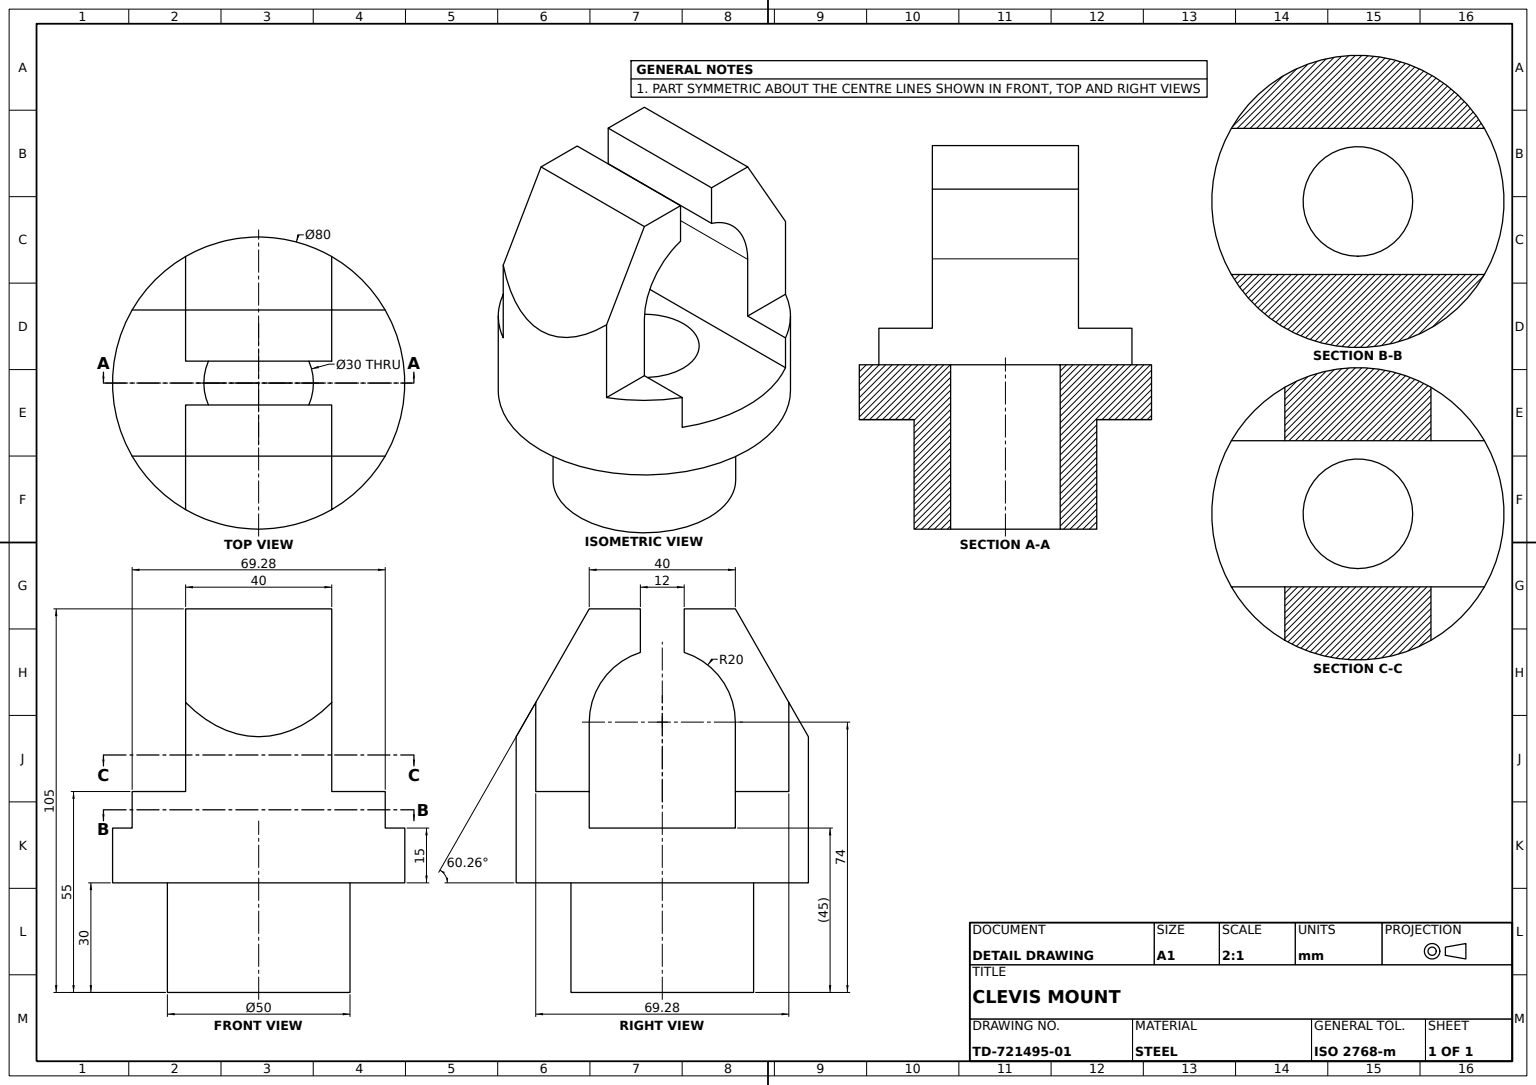
ISO-10303-21;
HEADER;
FILE_DESCRIPTION((''),'2;1');
FILE_NAME('','',(''),(''),'','','');
FILE_SCHEMA(('AUTOMOTIVE_DESIGN'));
ENDSEC;
DATA;
#1=APPLICATION_CONTEXT('');
#2=PRODUCT_CONTEXT('',#1,'mechanical');
#3=PRODUCT('','','',(#2));
#4=PRODUCT_DEFINITION_FORMATION('','',#3);
#5=PRODUCT_DEFINITION_CONTEXT('',#1,'design');
#6=PRODUCT_DEFINITION('','',#4,#5);
#7=PRODUCT_DEFINITION_SHAPE('','',#6);
#8=(LENGTH_UNIT()NAMED_UNIT(*)SI_UNIT(.MILLI.,.METRE.));
#9=(NAMED_UNIT(*)PLANE_ANGLE_UNIT()SI_UNIT($,.RADIAN.));
#10=(NAMED_UNIT(*)SI_UNIT($,.STERADIAN.)SOLID_ANGLE_UNIT());
#11=UNCERTAINTY_MEASURE_WITH_UNIT(LENGTH_MEASURE(0.005),#8,'distance_accuracy_value','');
#12=(GEOMETRIC_REPRESENTATION_CONTEXT(3)GLOBAL_UNCERTAINTY_ASSIGNED_CONTEXT((#11))GLOBAL_UNIT_ASSIGNED_CONTEXT((#8,#9,#10))REPRESENTATION_CONTEXT('',''));
#13=CARTESIAN_POINT('',(20.,34.641016,79.378222));
#14=VERTEX_POINT('',#13);
#15=CARTESIAN_POINT('',(20.,20.,105.));
#16=VERTEX_POINT('',#15);
#17=CARTESIAN_POINT('',(20.,60.307692,34.461538));
#18=DIRECTION('',(0.,-0.496138938,0.868243142));
#19=VECTOR('',#18,1000.);
#20=LINE('',#17,#19);
#21=EDGE_CURVE('',#14,#16,#20,.T.);
#22=ORIENTED_EDGE('',*,*,#21,.F.);
#23=CARTESIAN_POINT('',(-20.,34.641016,79.378222));
#24=VERTEX_POINT('',#23);
#25=CARTESIAN_POINT('',(0.,0.,140.));
#26=DIRECTION('',(0.,-0.868243142,-0.496138938));
#27=DIRECTION('',(0.,0.496138938,-0.868243142));
#28=AXIS2_PLACEMENT_3D('',#25,#26,#27);
#29=ELLIPSE('',#28,80.622577,40.);
#30=EDGE_CURVE('',#14,#24,#29,.F.);
#31=ORIENTED_EDGE('',*,*,#30,.T.);
#32=CARTESIAN_POINT('',(-20.,20.,105.));
#33=VERTEX_POINT('',#32);
#34=CARTESIAN_POINT('',(-20.,60.307692,34.461538));
#35=LINE('',#34,#19);
#36=EDGE_CURVE('',#24,#33,#35,.T.);
#37=ORIENTED_EDGE('',*,*,#36,.T.);
#38=CARTESIAN_POINT('',(50.,20.,105.));
#39=DIRECTION('',(-1.,0.,0.));
#40=VECTOR('',#39,1000.);
#41=LINE('',#38,#40);
#42=EDGE_CURVE('',#16,#33,#41,.T.);
#43=ORIENTED_EDGE('',*,*,#42,.F.);
#44=EDGE_LOOP('',(#22,#31,#37,#43));
#45=FACE_BOUND('',#44,.T.);
#46=CARTESIAN_POINT('',(50.,40.,70.));
#47=AXIS2_PLACEMENT_3D('',#46,#26,#27);
#48=PLANE('',#47);
#49=ADVANCED_FACE('',(#45),#48,.F.);
#50=CARTESIAN_POINT('',(34.641016,-20.,45.));
#51=VERTEX_POINT('',#50);
#52=CARTESIAN_POINT('',(34.641016,-20.,55.));
#53=VERTEX_POINT('',#52);
#54=CARTESIAN_POINT('',(34.641016,-20.,105.));
#55=DIRECTION('',(0.,0.,-1.));
#56=VECTOR('',#55,1000.);
#57=LINE('',#54,#56);
#58=EDGE_CURVE('',#51,#53,#57,.F.);
#59=ORIENTED_EDGE('',*,*,#58,.F.);
#60=CARTESIAN_POINT('',(-34.641016,-20.,45.));
#61=VERTEX_POINT('',#60);
#62=CARTESIAN_POINT('',(70.,-20.,45.));
#63=LINE('',#62,#40);
#64=EDGE_CURVE('',#61,#51,#63,.F.);
#65=ORIENTED_EDGE('',*,*,#64,.F.);
#66=CARTESIAN_POINT('',(-34.641016,-20.,55.));
#67=VERTEX_POINT('',#66);
#68=CARTESIAN_POINT('',(-34.641016,-20.,105.));
#69=LINE('',#68,#56);
#70=EDGE_CURVE('',#67,#61,#69,.T.);
#71=ORIENTED_EDGE('',*,*,#70,.F.);
#72=CARTESIAN_POINT('',(-20.,-20.,55.));
#73=VERTEX_POINT('',#72);
#74=CARTESIAN_POINT('',(70.,-20.,55.));
#75=DIRECTION('',(1.,0.,0.));
#76=VECTOR('',#75,1000.);
#77=LINE('',#74,#76);
#78=EDGE_CURVE('',#67,#73,#77,.T.);
#79=ORIENTED_EDGE('',*,*,#78,.T.);
#80=CARTESIAN_POINT('',(-20.,-20.,74.));
#81=VERTEX_POINT('',#80);
#82=DIRECTION('',(0.,0.,1.));
#83=VECTOR('',#82,1000.);
#84=LINE('',#80,#83);
#85=EDGE_CURVE('',#73,#81,#84,.T.);
#86=ORIENTED_EDGE('',*,*,#85,.T.);
#87=CARTESIAN_POINT('',(20.,-20.,74.));
#88=VERTEX_POINT('',#87);
#89=CARTESIAN_POINT('',(70.,-20.,74.));
#90=LINE('',#89,#40);
#91=EDGE_CURVE('',#81,#88,#90,.F.);
#92=ORIENTED_EDGE('',*,*,#91,.T.);
#93=CARTESIAN_POINT('',(20.,-20.,55.));
#94=VERTEX_POINT('',#93);
#95=LINE('',#87,#83);
#96=EDGE_CURVE('',#94,#88,#95,.T.);
#97=ORIENTED_EDGE('',*,*,#96,.F.);
#98=LINE('',#74,#40);
#99=EDGE_CURVE('',#53,#94,#98,.T.);
#100=ORIENTED_EDGE('',*,*,#99,.F.);
#101=EDGE_LOOP('',(#59,#65,#71,#79,#86,#92,#97,#100));
#102=FACE_BOUND('',#101,.T.);
#103=DIRECTION('',(0.,1.,0.));
#104=AXIS2_PLACEMENT_3D('',#89,#103,#82);
#105=PLANE('',#104);
#106=ADVANCED_FACE('',(#102),#105,.T.);
#107=CARTESIAN_POINT('',(-34.641016,20.,45.));
#108=VERTEX_POINT('',#107);
#109=CARTESIAN_POINT('',(0.,0.,45.));
#110=DIRECTION('',(0.,-1.,0.));
#111=AXIS2_PLACEMENT_3D('',#109,#82,#110);
#112=CIRCLE('',#111,40.);
#113=EDGE_CURVE('',#61,#108,#112,.F.);
#114=ORIENTED_EDGE('',*,*,#113,.F.);
#115=ORIENTED_EDGE('',*,*,#64,.T.);
#116=CARTESIAN_POINT('',(34.641016,20.,45.));
#117=VERTEX_POINT('',#116);
#118=EDGE_CURVE('',#117,#51,#112,.F.);
#119=ORIENTED_EDGE('',*,*,#118,.F.);
#120=CARTESIAN_POINT('',(70.,20.,45.));
#121=LINE('',#120,#40);
#122=EDGE_CURVE('',#108,#117,#121,.F.);
#123=ORIENTED_EDGE('',*,*,#122,.F.);
#124=EDGE_LOOP('',(#114,#115,#119,#123));
#125=FACE_BOUND('',#124,.T.);
#126=CARTESIAN_POINT('',(0.,-15.,45.));
#127=VERTEX_POINT('',#126);
#128=CIRCLE('',#111,15.);
#129=EDGE_CURVE('',#127,#127,#128,.T.);
#130=ORIENTED_EDGE('',*,*,#129,.F.);
#131=EDGE_LOOP('',(#130));
#132=FACE_BOUND('',#131,.T.);
#133=AXIS2_PLACEMENT_3D('',#62,#82,#110);
#134=PLANE('',#133);
#135=ADVANCED_FACE('',(#125,#132),#134,.T.);
#136=CARTESIAN_POINT('',(20.,-34.641016,79.378222));
#137=VERTEX_POINT('',#136);
#138=CARTESIAN_POINT('',(20.,-20.,105.));
#139=VERTEX_POINT('',#138);
#140=CARTESIAN_POINT('',(20.,-60.307692,34.461538));
#141=DIRECTION('',(0.,0.496138938,0.868243142));
#142=VECTOR('',#141,1000.);
#143=LINE('',#140,#142);
#144=EDGE_CURVE('',#137,#139,#143,.T.);
#145=ORIENTED_EDGE('',*,*,#144,.T.);
#146=CARTESIAN_POINT('',(-20.,-20.,105.));
#147=VERTEX_POINT('',#146);
#148=CARTESIAN_POINT('',(50.,-20.,105.));
#149=LINE('',#148,#40);
#150=EDGE_CURVE('',#139,#147,#149,.T.);
#151=ORIENTED_EDGE('',*,*,#150,.T.);
#152=CARTESIAN_POINT('',(-20.,-34.641016,79.378222));
#153=VERTEX_POINT('',#152);
#154=CARTESIAN_POINT('',(-20.,-60.307692,34.461538));
#155=LINE('',#154,#142);
#156=EDGE_CURVE('',#153,#147,#155,.T.);
#157=ORIENTED_EDGE('',*,*,#156,.F.);
#158=DIRECTION('',(0.,-0.868243142,0.496138938));
#159=DIRECTION('',(0.,-0.496138938,-0.868243142));
#160=AXIS2_PLACEMENT_3D('',#25,#158,#159);
#161=ELLIPSE('',#160,80.622577,40.);
#162=EDGE_CURVE('',#137,#153,#161,.F.);
#163=ORIENTED_EDGE('',*,*,#162,.F.);
#164=EDGE_LOOP('',(#145,#151,#157,#163));
#165=FACE_BOUND('',#164,.T.);
#166=CARTESIAN_POINT('',(50.,-40.,70.));
#167=AXIS2_PLACEMENT_3D('',#166,#158,#159);
#168=PLANE('',#167);
#169=ADVANCED_FACE('',(#165),#168,.T.);
#170=CARTESIAN_POINT('',(-34.641016,20.,55.));
#171=VERTEX_POINT('',#170);
#172=CARTESIAN_POINT('',(-34.641016,20.,105.));
#173=LINE('',#172,#56);
#174=EDGE_CURVE('',#108,#171,#173,.F.);
#175=ORIENTED_EDGE('',*,*,#174,.F.);
#176=ORIENTED_EDGE('',*,*,#122,.T.);
#177=CARTESIAN_POINT('',(34.641016,20.,55.));
#178=VERTEX_POINT('',#177);
#179=CARTESIAN_POINT('',(34.641016,20.,105.));
#180=LINE('',#179,#56);
#181=EDGE_CURVE('',#178,#117,#180,.T.);
#182=ORIENTED_EDGE('',*,*,#181,.F.);
#183=CARTESIAN_POINT('',(20.,20.,55.));
#184=VERTEX_POINT('',#183);
#185=CARTESIAN_POINT('',(70.,20.,55.));
#186=LINE('',#185,#76);
#187=EDGE_CURVE('',#184,#178,#186,.T.);
#188=ORIENTED_EDGE('',*,*,#187,.F.);
#189=CARTESIAN_POINT('',(20.,20.,74.));
#190=VERTEX_POINT('',#189);
#191=CARTESIAN_POINT('',(20.,20.,45.));
#192=LINE('',#191,#56);
#193=EDGE_CURVE('',#190,#184,#192,.T.);
#194=ORIENTED_EDGE('',*,*,#193,.F.);
#195=CARTESIAN_POINT('',(-20.,20.,74.));
#196=VERTEX_POINT('',#195);
#197=CARTESIAN_POINT('',(70.,20.,74.));
#198=LINE('',#197,#40);
#199=EDGE_CURVE('',#196,#190,#198,.F.);
#200=ORIENTED_EDGE('',*,*,#199,.F.);
#201=CARTESIAN_POINT('',(-20.,20.,55.));
#202=VERTEX_POINT('',#201);
#203=CARTESIAN_POINT('',(-20.,20.,45.));
#204=LINE('',#203,#56);
#205=EDGE_CURVE('',#196,#202,#204,.T.);
#206=ORIENTED_EDGE('',*,*,#205,.T.);
#207=LINE('',#185,#40);
#208=EDGE_CURVE('',#202,#171,#207,.T.);
#209=ORIENTED_EDGE('',*,*,#208,.T.);
#210=EDGE_LOOP('',(#175,#176,#182,#188,#194,#200,#206,#209));
#211=FACE_BOUND('',#210,.T.);
#212=AXIS2_PLACEMENT_3D('',#120,#110,#55);
#213=PLANE('',#212);
#214=ADVANCED_FACE('',(#211),#213,.T.);
#215=CARTESIAN_POINT('',(-20.,-6.,105.));
#216=VERTEX_POINT('',#215);
#217=CARTESIAN_POINT('',(-20.,-6.,93.078784));
#218=VERTEX_POINT('',#217);
#219=CARTESIAN_POINT('',(-20.,-6.,135.));
#220=LINE('',#219,#56);
#221=EDGE_CURVE('',#216,#218,#220,.T.);
#222=ORIENTED_EDGE('',*,*,#221,.F.);
#223=CARTESIAN_POINT('',(20.,-6.,105.));
#224=VERTEX_POINT('',#223);
#225=CARTESIAN_POINT('',(0.,-6.,105.));
#226=LINE('',#225,#40);
#227=EDGE_CURVE('',#224,#216,#226,.T.);
#228=ORIENTED_EDGE('',*,*,#227,.F.);
#229=CARTESIAN_POINT('',(20.,-6.,93.078784));
#230=VERTEX_POINT('',#229);
#231=CARTESIAN_POINT('',(20.,-6.,135.));
#232=LINE('',#231,#56);
#233=EDGE_CURVE('',#224,#230,#232,.T.);
#234=ORIENTED_EDGE('',*,*,#233,.T.);
#235=CARTESIAN_POINT('',(70.,-6.,93.078784));
#236=LINE('',#235,#40);
#237=EDGE_CURVE('',#230,#218,#236,.T.);
#238=ORIENTED_EDGE('',*,*,#237,.T.);
#239=EDGE_LOOP('',(#222,#228,#234,#238));
#240=FACE_BOUND('',#239,.T.);
#241=AXIS2_PLACEMENT_3D('',#231,#110,#55);
#242=PLANE('',#241);
#243=ADVANCED_FACE('',(#240),#242,.F.);
#244=CARTESIAN_POINT('',(20.,6.,93.078784));
#245=VERTEX_POINT('',#244);
#246=CARTESIAN_POINT('',(20.,0.,74.));
#247=AXIS2_PLACEMENT_3D('',#246,#39,#82);
#248=CIRCLE('',#247,20.);
#249=EDGE_CURVE('',#245,#190,#248,.T.);
#250=ORIENTED_EDGE('',*,*,#249,.T.);
#251=ORIENTED_EDGE('',*,*,#193,.T.);
#252=CARTESIAN_POINT('',(20.,34.641016,55.));
#253=VERTEX_POINT('',#252);
#254=CARTESIAN_POINT('',(20.,37.310673,55.));
#255=VECTOR('',#110,1000.);
#256=LINE('',#254,#255);
#257=EDGE_CURVE('',#184,#253,#256,.F.);
#258=ORIENTED_EDGE('',*,*,#257,.T.);
#259=CARTESIAN_POINT('',(20.,34.641016,105.));
#260=LINE('',#259,#56);
#261=EDGE_CURVE('',#253,#14,#260,.F.);
#262=ORIENTED_EDGE('',*,*,#261,.T.);
#263=ORIENTED_EDGE('',*,*,#21,.T.);
#264=CARTESIAN_POINT('',(20.,6.,105.));
#265=VERTEX_POINT('',#264);
#266=CARTESIAN_POINT('',(20.,-35.929094,105.));
#267=VECTOR('',#103,1000.);
#268=LINE('',#266,#267);
#269=EDGE_CURVE('',#265,#16,#268,.T.);
#270=ORIENTED_EDGE('',*,*,#269,.F.);
#271=CARTESIAN_POINT('',(20.,6.,135.));
#272=LINE('',#271,#56);
#273=EDGE_CURVE('',#265,#245,#272,.T.);
#274=ORIENTED_EDGE('',*,*,#273,.T.);
#275=EDGE_LOOP('',(#250,#251,#258,#262,#263,#270,#274));
#276=FACE_BOUND('',#275,.T.);
#277=CARTESIAN_POINT('',(20.,0.,0.));
#278=AXIS2_PLACEMENT_3D('',#277,#39,#82);
#279=PLANE('',#278);
#280=ADVANCED_FACE('',(#276),#279,.F.);
#281=CARTESIAN_POINT('',(0.,0.,55.));
#282=AXIS2_PLACEMENT_3D('',#281,#55,#103);
#283=CIRCLE('',#282,40.);
#284=EDGE_CURVE('',#178,#253,#283,.F.);
#285=ORIENTED_EDGE('',*,*,#284,.T.);
#286=ORIENTED_EDGE('',*,*,#257,.F.);
#287=ORIENTED_EDGE('',*,*,#187,.T.);
#288=EDGE_LOOP('',(#285,#286,#287));
#289=FACE_BOUND('',#288,.T.);
#290=CARTESIAN_POINT('',(56.,37.310673,55.));
#291=AXIS2_PLACEMENT_3D('',#290,#55,#103);
#292=PLANE('',#291);
#293=ADVANCED_FACE('',(#289),#292,.F.);
#294=CARTESIAN_POINT('',(25.,0.,0.));
#295=VERTEX_POINT('',#294);
#296=CARTESIAN_POINT('',(0.,0.,0.));
#297=AXIS2_PLACEMENT_3D('',#296,#55,#75);
#298=CIRCLE('',#297,25.);
#299=EDGE_CURVE('',#295,#295,#298,.T.);
#300=ORIENTED_EDGE('',*,*,#299,.F.);
#301=EDGE_LOOP('',(#300));
#302=FACE_BOUND('',#301,.T.);
#303=CARTESIAN_POINT('',(25.,0.,30.));
#304=VERTEX_POINT('',#303);
#305=CARTESIAN_POINT('',(0.,0.,30.));
#306=AXIS2_PLACEMENT_3D('',#305,#55,#75);
#307=CIRCLE('',#306,25.);
#308=EDGE_CURVE('',#304,#304,#307,.T.);
#309=ORIENTED_EDGE('',*,*,#308,.T.);
#310=EDGE_LOOP('',(#309));
#311=FACE_BOUND('',#310,.T.);
#312=AXIS2_PLACEMENT_3D('',#305,#55,#39);
#313=CYLINDRICAL_SURFACE('',#312,25.);
#314=ADVANCED_FACE('',(#302,#311),#313,.T.);
#315=ORIENTED_EDGE('',*,*,#99,.T.);
#316=CARTESIAN_POINT('',(20.,-34.641016,55.));
#317=VERTEX_POINT('',#316);
#318=EDGE_CURVE('',#317,#94,#256,.F.);
#319=ORIENTED_EDGE('',*,*,#318,.F.);
#320=EDGE_CURVE('',#317,#53,#283,.F.);
#321=ORIENTED_EDGE('',*,*,#320,.T.);
#322=EDGE_LOOP('',(#315,#319,#321));
#323=FACE_BOUND('',#322,.T.);
#324=ADVANCED_FACE('',(#323),#292,.F.);
#325=ORIENTED_EDGE('',*,*,#249,.F.);
#326=CARTESIAN_POINT('',(-20.,6.,93.078784));
#327=VERTEX_POINT('',#326);
#328=CARTESIAN_POINT('',(70.,6.,93.078784));
#329=LINE('',#328,#40);
#330=EDGE_CURVE('',#327,#245,#329,.F.);
#331=ORIENTED_EDGE('',*,*,#330,.F.);
#332=CARTESIAN_POINT('',(-20.,0.,74.));
#333=AXIS2_PLACEMENT_3D('',#332,#39,#82);
#334=CIRCLE('',#333,20.);
#335=EDGE_CURVE('',#327,#196,#334,.T.);
#336=ORIENTED_EDGE('',*,*,#335,.T.);
#337=ORIENTED_EDGE('',*,*,#199,.T.);
#338=EDGE_LOOP('',(#325,#331,#336,#337));
#339=FACE_BOUND('',#338,.T.);
#340=CARTESIAN_POINT('',(70.,0.,74.));
#341=AXIS2_PLACEMENT_3D('',#340,#39,#82);
#342=CYLINDRICAL_SURFACE('',#341,20.);
#343=ADVANCED_FACE('',(#339),#342,.F.);
#344=EDGE_CURVE('',#81,#218,#334,.T.);
#345=ORIENTED_EDGE('',*,*,#344,.T.);
#346=ORIENTED_EDGE('',*,*,#237,.F.);
#347=EDGE_CURVE('',#88,#230,#248,.T.);
#348=ORIENTED_EDGE('',*,*,#347,.F.);
#349=ORIENTED_EDGE('',*,*,#91,.F.);
#350=EDGE_LOOP('',(#345,#346,#348,#349));
#351=FACE_BOUND('',#350,.T.);
#352=ADVANCED_FACE('',(#351),#342,.F.);
#353=ORIENTED_EDGE('',*,*,#221,.T.);
#354=ORIENTED_EDGE('',*,*,#344,.F.);
#355=ORIENTED_EDGE('',*,*,#85,.F.);
#356=CARTESIAN_POINT('',(-20.,-34.641016,55.));
#357=VERTEX_POINT('',#356);
#358=CARTESIAN_POINT('',(-20.,37.310673,55.));
#359=LINE('',#358,#255);
#360=EDGE_CURVE('',#357,#73,#359,.F.);
#361=ORIENTED_EDGE('',*,*,#360,.F.);
#362=CARTESIAN_POINT('',(-20.,-34.641016,105.));
#363=LINE('',#362,#56);
#364=EDGE_CURVE('',#153,#357,#363,.T.);
#365=ORIENTED_EDGE('',*,*,#364,.F.);
#366=ORIENTED_EDGE('',*,*,#156,.T.);
#367=CARTESIAN_POINT('',(-20.,-35.929094,105.));
#368=LINE('',#367,#267);
#369=EDGE_CURVE('',#147,#216,#368,.T.);
#370=ORIENTED_EDGE('',*,*,#369,.T.);
#371=EDGE_LOOP('',(#353,#354,#355,#361,#365,#366,#370));
#372=FACE_BOUND('',#371,.T.);
#373=CARTESIAN_POINT('',(-20.,0.,0.));
#374=AXIS2_PLACEMENT_3D('',#373,#39,#82);
#375=PLANE('',#374);
#376=ADVANCED_FACE('',(#372),#375,.T.);
#377=CARTESIAN_POINT('',(-20.,6.,105.));
#378=VERTEX_POINT('',#377);
#379=CARTESIAN_POINT('',(0.,6.,105.));
#380=LINE('',#379,#76);
#381=EDGE_CURVE('',#378,#265,#380,.T.);
#382=ORIENTED_EDGE('',*,*,#381,.F.);
#383=CARTESIAN_POINT('',(-20.,6.,135.));
#384=LINE('',#383,#56);
#385=EDGE_CURVE('',#378,#327,#384,.T.);
#386=ORIENTED_EDGE('',*,*,#385,.T.);
#387=ORIENTED_EDGE('',*,*,#330,.T.);
#388=ORIENTED_EDGE('',*,*,#273,.F.);
#389=EDGE_LOOP('',(#382,#386,#387,#388));
#390=FACE_BOUND('',#389,.T.);
#391=AXIS2_PLACEMENT_3D('',#383,#103,#82);
#392=PLANE('',#391);
#393=ADVANCED_FACE('',(#390),#392,.F.);
#394=ORIENTED_EDGE('',*,*,#118,.T.);
#395=ORIENTED_EDGE('',*,*,#58,.T.);
#396=ORIENTED_EDGE('',*,*,#320,.F.);
#397=CARTESIAN_POINT('',(20.,-34.641016,105.));
#398=LINE('',#397,#56);
#399=EDGE_CURVE('',#137,#317,#398,.T.);
#400=ORIENTED_EDGE('',*,*,#399,.F.);
#401=ORIENTED_EDGE('',*,*,#162,.T.);
#402=ORIENTED_EDGE('',*,*,#364,.T.);
#403=AXIS2_PLACEMENT_3D('',#281,#82,#110);
#404=CIRCLE('',#403,40.);
#405=EDGE_CURVE('',#357,#67,#404,.F.);
#406=ORIENTED_EDGE('',*,*,#405,.T.);
#407=ORIENTED_EDGE('',*,*,#70,.T.);
#408=ORIENTED_EDGE('',*,*,#113,.T.);
#409=ORIENTED_EDGE('',*,*,#174,.T.);
#410=CARTESIAN_POINT('',(-20.,34.641016,55.));
#411=VERTEX_POINT('',#410);
#412=EDGE_CURVE('',#171,#411,#404,.F.);
#413=ORIENTED_EDGE('',*,*,#412,.T.);
#414=CARTESIAN_POINT('',(-20.,34.641016,105.));
#415=LINE('',#414,#56);
#416=EDGE_CURVE('',#411,#24,#415,.F.);
#417=ORIENTED_EDGE('',*,*,#416,.T.);
#418=ORIENTED_EDGE('',*,*,#30,.F.);
#419=ORIENTED_EDGE('',*,*,#261,.F.);
#420=ORIENTED_EDGE('',*,*,#284,.F.);
#421=ORIENTED_EDGE('',*,*,#181,.T.);
#422=EDGE_LOOP('',(#394,#395,#396,#400,#401,#402,#406,#407,#408,#409,#413,#417,#418,#419,#420,#421));
#423=FACE_BOUND('',#422,.T.);
#424=CARTESIAN_POINT('',(40.,0.,30.));
#425=VERTEX_POINT('',#424);
#426=CIRCLE('',#306,40.);
#427=EDGE_CURVE('',#425,#425,#426,.T.);
#428=ORIENTED_EDGE('',*,*,#427,.F.);
#429=EDGE_LOOP('',(#428));
#430=FACE_BOUND('',#429,.T.);
#431=CARTESIAN_POINT('',(0.,0.,105.));
#432=AXIS2_PLACEMENT_3D('',#431,#55,#39);
#433=CYLINDRICAL_SURFACE('',#432,40.);
#434=ADVANCED_FACE('',(#423,#430),#433,.T.);
#435=CARTESIAN_POINT('',(15.,0.,0.));
#436=VERTEX_POINT('',#435);
#437=AXIS2_PLACEMENT_3D('',#296,#82,#75);
#438=CIRCLE('',#437,15.);
#439=EDGE_CURVE('',#436,#436,#438,.T.);
#440=ORIENTED_EDGE('',*,*,#439,.T.);
#441=EDGE_LOOP('',(#440));
#442=FACE_BOUND('',#441,.T.);
#443=ORIENTED_EDGE('',*,*,#299,.T.);
#444=EDGE_LOOP('',(#443));
#445=FACE_BOUND('',#444,.T.);
#446=AXIS2_PLACEMENT_3D('',#296,#55,#39);
#447=PLANE('',#446);
#448=ADVANCED_FACE('',(#442,#445),#447,.T.);
#449=ORIENTED_EDGE('',*,*,#439,.F.);
#450=EDGE_LOOP('',(#449));
#451=FACE_BOUND('',#450,.T.);
#452=ORIENTED_EDGE('',*,*,#129,.T.);
#453=EDGE_LOOP('',(#452));
#454=FACE_BOUND('',#453,.T.);
#455=CYLINDRICAL_SURFACE('',#437,15.);
#456=ADVANCED_FACE('',(#451,#454),#455,.F.);
#457=ORIENTED_EDGE('',*,*,#144,.F.);
#458=ORIENTED_EDGE('',*,*,#399,.T.);
#459=ORIENTED_EDGE('',*,*,#318,.T.);
#460=ORIENTED_EDGE('',*,*,#96,.T.);
#461=ORIENTED_EDGE('',*,*,#347,.T.);
#462=ORIENTED_EDGE('',*,*,#233,.F.);
#463=EDGE_CURVE('',#139,#224,#268,.T.);
#464=ORIENTED_EDGE('',*,*,#463,.F.);
#465=EDGE_LOOP('',(#457,#458,#459,#460,#461,#462,#464));
#466=FACE_BOUND('',#465,.T.);
#467=ADVANCED_FACE('',(#466),#279,.F.);
#468=ORIENTED_EDGE('',*,*,#308,.F.);
#469=EDGE_LOOP('',(#468));
#470=FACE_BOUND('',#469,.T.);
#471=ORIENTED_EDGE('',*,*,#427,.T.);
#472=EDGE_LOOP('',(#471));
#473=FACE_BOUND('',#472,.T.);
#474=PLANE('',#312);
#475=ADVANCED_FACE('',(#470,#473),#474,.T.);
#476=ORIENTED_EDGE('',*,*,#42,.T.);
#477=EDGE_CURVE('',#378,#33,#368,.T.);
#478=ORIENTED_EDGE('',*,*,#477,.F.);
#479=ORIENTED_EDGE('',*,*,#381,.T.);
#480=ORIENTED_EDGE('',*,*,#269,.T.);
#481=EDGE_LOOP('',(#476,#478,#479,#480));
#482=FACE_BOUND('',#481,.T.);
#483=PLANE('',#432);
#484=ADVANCED_FACE('',(#482),#483,.F.);
#485=ORIENTED_EDGE('',*,*,#208,.F.);
#486=EDGE_CURVE('',#202,#411,#359,.F.);
#487=ORIENTED_EDGE('',*,*,#486,.T.);
#488=ORIENTED_EDGE('',*,*,#412,.F.);
#489=EDGE_LOOP('',(#485,#487,#488));
#490=FACE_BOUND('',#489,.T.);
#491=CARTESIAN_POINT('',(-56.,37.310673,55.));
#492=AXIS2_PLACEMENT_3D('',#491,#82,#110);
#493=PLANE('',#492);
#494=ADVANCED_FACE('',(#490),#493,.T.);
#495=ORIENTED_EDGE('',*,*,#477,.T.);
#496=ORIENTED_EDGE('',*,*,#36,.F.);
#497=ORIENTED_EDGE('',*,*,#416,.F.);
#498=ORIENTED_EDGE('',*,*,#486,.F.);
#499=ORIENTED_EDGE('',*,*,#205,.F.);
#500=ORIENTED_EDGE('',*,*,#335,.F.);
#501=ORIENTED_EDGE('',*,*,#385,.F.);
#502=EDGE_LOOP('',(#495,#496,#497,#498,#499,#500,#501));
#503=FACE_BOUND('',#502,.T.);
#504=ADVANCED_FACE('',(#503),#375,.T.);
#505=ORIENTED_EDGE('',*,*,#150,.F.);
#506=ORIENTED_EDGE('',*,*,#463,.T.);
#507=ORIENTED_EDGE('',*,*,#227,.T.);
#508=ORIENTED_EDGE('',*,*,#369,.F.);
#509=EDGE_LOOP('',(#505,#506,#507,#508));
#510=FACE_BOUND('',#509,.T.);
#511=ADVANCED_FACE('',(#510),#483,.F.);
#512=ORIENTED_EDGE('',*,*,#405,.F.);
#513=ORIENTED_EDGE('',*,*,#360,.T.);
#514=ORIENTED_EDGE('',*,*,#78,.F.);
#515=EDGE_LOOP('',(#512,#513,#514));
#516=FACE_BOUND('',#515,.T.);
#517=ADVANCED_FACE('',(#516),#493,.T.);
#518=CLOSED_SHELL('',(#49,#106,#135,#169,#214,#243,#280,#293,#314,#324,#343,#352,#376,#393,#434,#448,#456,#467,#475,#484,#494,#504,#511,#517));
#519=MANIFOLD_SOLID_BREP('',#518);
#520=ADVANCED_BREP_SHAPE_REPRESENTATION('',(#519),#12);
#521=SHAPE_DEFINITION_REPRESENTATION(#7,#520);
ENDSEC;
END-ISO-10303-21;
